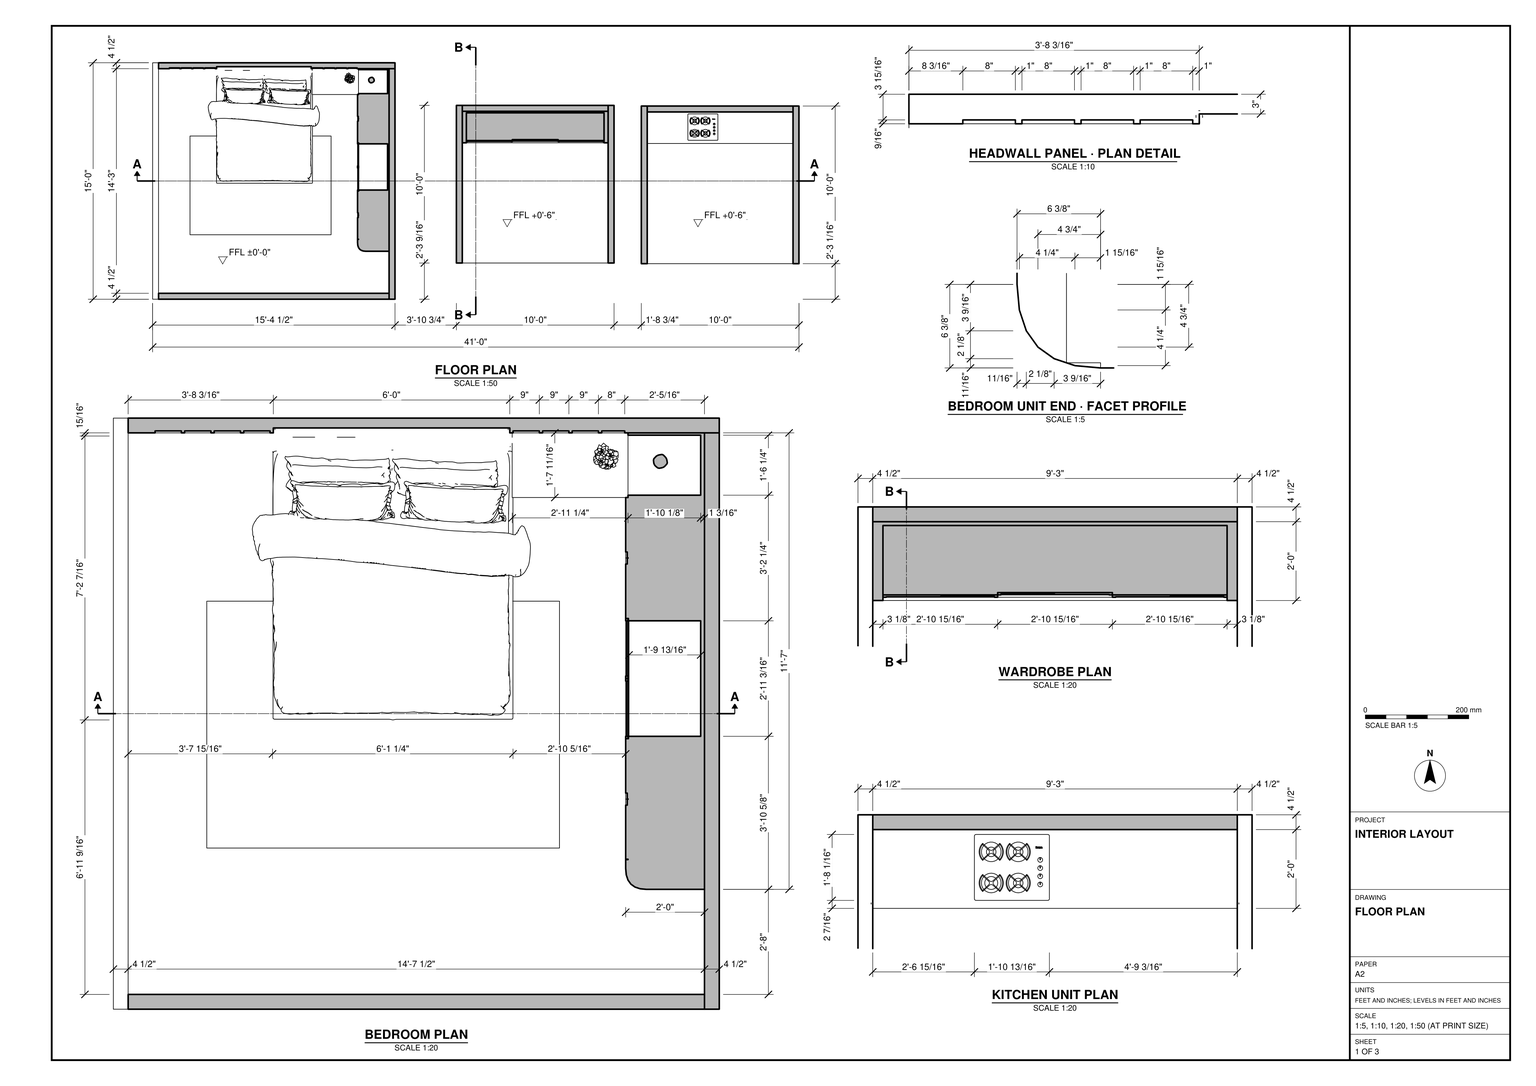
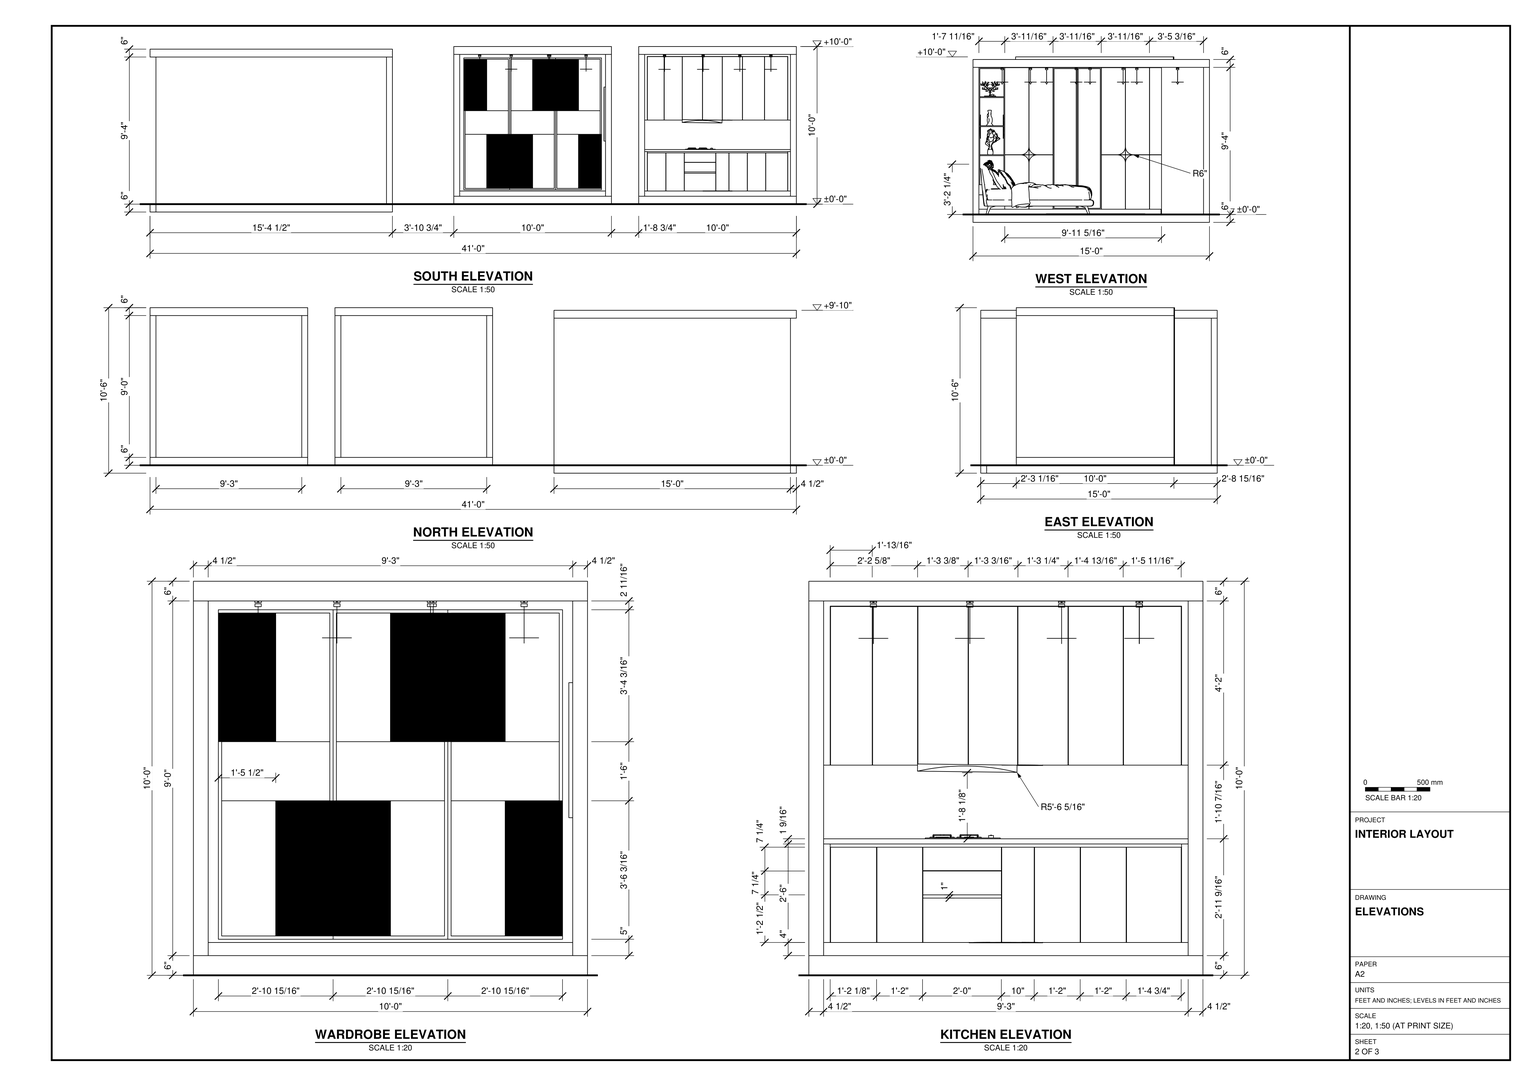
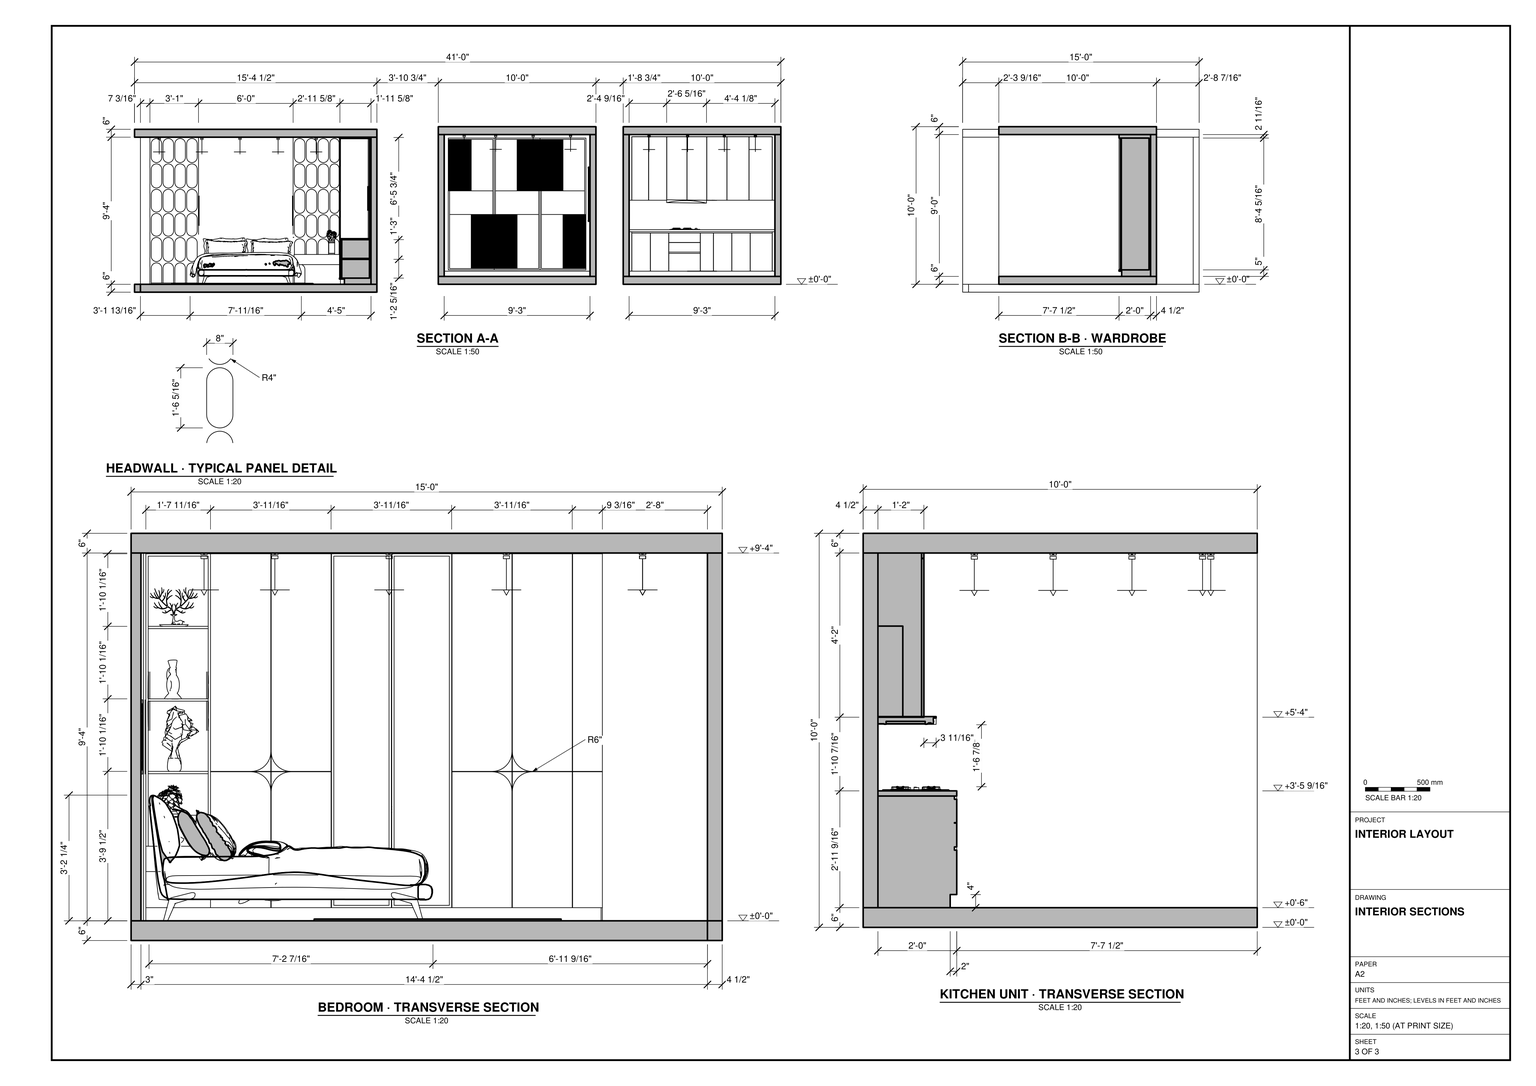
Build the interior layout in SketchUp from task_files/diagram_01.pdf. Work in feet and inches. The overall model is 41'-0" long, 15'-0" deep and 10'-6" high. Use the bedroom finished floor at ±0'-0" as the storey datum. Set the wardrobe and kitchen finished floors at +0'-6"; these are raised bays on the same storey.

Place the 15'-4 1/2" wide bedroom on the left, the wardrobe in the middle and the kitchen on the right. Follow the floor plan for the gaps and setbacks between bays. Form the 4 1/2" walls and 6" floor and overhead slabs, leaving the open faces as drawn. In the bedroom, position the bed against the headwall between the fields of rounded panels. Reproduce the side-wall storage unit with its display shelves, divided fronts and shaped end. Use the enlarged plans and elevations to lay out the wardrobe fronts and the kitchen counter, drawers and upper cabinets. Align the hood with the cooktop.

Decor and loose items, including the rug, cushions, shelf objects, lights and appliances, may be any suitable library components placed as shown. Keep shell elements and individual furniture and joinery pieces in separate groups or components, and use components for repeated parts. Save one SketchUp model as output_files/bedroom_wardrobe_and_kitchen_bays.skp.

# SketchUp Ruby script. Lengths in inches.
U = 1.inch
M = Sketchup.active_model
def pt(a) = Geom::Point3d.new(a.map { |v| v * U })
def face(e, loops, mat)
  f = e.add_face(loops[0].map { |a| pt(a) })
  loops[1..].each { |l| e.add_face(l.map { |a| pt(a) }).erase! }
  f.material = f.back_material = mat if mat
  f
end
# faces: each face lists its corners as indices into pts; further lists are holes
def faces(e, pts, list, mat = nil) = list.each { |f| face(e, (f[0].is_a?(Array) ? f : [f]).map { |l| l.map { |i| pts[i] } }, mat) }
# xy, xz, yz: faces in a plane at the given z, y or x. An outline is a flat list of corners, or four numbers for a rectangle; further outlines are holes
def ring(l) = l.size == 4 ? [[l[0], l[1]], [l[2], l[1]], [l[2], l[3]], [l[0], l[3]]] : l.each_slice(2).to_a
def flat(e, list, mat, &to3) = list.each { |f| face(e, (f[0].is_a?(Array) ? f : [f]).map { |l| ring(l).map { |u, v| to3.(u, v) } }, mat) }
def xy(e, z, list, mat = nil) = flat(e, list, mat) { |x, y| [x, y, z] }
def xz(e, y, list, mat = nil) = flat(e, list, mat) { |x, z| [x, y, z] }
def yz(e, x, list, mat = nil) = flat(e, list, mat) { |y, z| [x, y, z] }
def lines(e, pts, list) = list.each { |a, b| e.add_line(pt(pts[a]), pt(pts[b])) }
# prism: a flat outline (further loops are holes) pulled along v
def prism(e, loops, v, mat = nil)
  f = face(e, loops, mat); d = Geom::Vector3d.new(v.map { |x| x * U })
  f.pushpull(f.normal.samedirection?(d) ? d.length : -d.length)
end
def box(e, o, s, mat = nil) = prism(e, [[o, [o[0] + s[0], o[1], o[2]], [o[0] + s[0], o[1] + s[1], o[2]], [o[0], o[1] + s[1], o[2]]]], [0, 0, s[2]], mat)
def at(x, y, z, deg = 0) = Geom::Transformation.translation(pt([x, y, z])) * Geom::Transformation.rotation(ORIGIN, Z_AXIS, deg.degrees)
def axes(o, x, y, z) = Geom::Transformation.new([*x, 0, *y, 0, *z, 0, *pt(o).to_a, 1])
def part(name) = M.definitions.add(name)
# library, detail: a bought-in or finely detailed component or shape, given as its bounding box
def library(name, o, s) = part(name).tap { |d| box(d.entities, o, s) }
def detail(e, o, s) = box(e.add_group.entities, o, s)
def put(e, d, t, mat = nil) = e.add_instance(d, t).tap { |i| i.material = mat if mat }
def group(e, t, mat = nil) = e.add_group.tap { |g| g.transformation = t; g.material = mat if mat }.entities
root = M.entities
M.materials.add("Oak Veneered MDF (VY2JTJ)").color = [209, 167, 120]
M.materials.add("Oak Veneered MDF (Z561KV)").color = [209, 167, 120]
M.materials.add("Sublime-3029-Pacifique-Glamour-or-Glamorous-Pacific-4K").color = [0, 52, 63]
M.materials.add("Teddy_BookCover").color = [245, 235, 215]
M.materials.add("Teddy_HairLight").color = [51, 36, 26]
M.materials.add("[Color M00]").color = [255, 255, 255]
M.materials["[Color M00]"].alpha = 0.43
M.materials.add("[Color M00]1").color = [255, 255, 255]
M.materials.add("[Color M09]").color = [0, 0, 0]
M.materials.add("[Translucent Glass Gray]").color = [128, 128, 128]
M.materials["[Translucent Glass Gray]"].alpha = 0.5
c1 = library("Спалня Венид",[0.07,-0.07,0],[84.71,86.8,39])
c2 = part("Area rug")
box(c2.entities,[0,0,0],[55.12,78.74,0.39])
c3 = part("Group56\#1")
p = [[0,0,0],[0,0,-43.71],[-13.13,0,-43.71],[85.5,-56,0],[-85.5,-56,0],[85.5,56,0],
  [85.5,0,0],[-85.5,56,0],[13.13,0,-43.71],[-85.5,0,0],[0,0,-70.75]]
lines(c3.entities,p,[[0,1],[1,2],[3,4],[5,6],[7,5],[1,8],[9,0],[0,6],[8,10],[4,9],[6,3],[2,10],
  [9,7]])
c4 = part("Rectangle Light")
put(c4.entities,c3,at(0,0,0))
c5 = library("Interior Props 221 030",[-2.57,-3.63,-0.04],[5.13,7.27,11.89])
c6 = library("Decorative Jar 83-09",[-5.58,-3.02,0],[11.21,6.04,13.74])
c7 = library("Decorative Deer 97-30",[-7.23,-2.03,0],[14.46,4,11.8125])
c8 = library("Interior Plant 273 003 001",[-15.3,-29.38,0],[45.32,44.44,78.66])
c9 = library("Potted Basil 50-07",[-3.85,-3.53,0.03],[7.56,8,18.65])
c10 = library("2-TABLE DE CUISSON CLC2",[-11.42,-10.04,0],[22.84,20.08,1.26])
c11 = library("5-HOTTE ASPIRANTE CLC2",[-15.16,-17.72,-0.29],[30.34,17.72,30.09])
c12 = library("Group\#2",[0,0,0],[180,4.5,112])
c13 = library("Group\#4",[-10.5625,9.18,0],[58.5625,139.01,111.76])
c14 = library("Group\#28",[-3.45,-3.45,-12.01],[8.9,8.9,12.86])
c15 = part("Group\#31")
box(c15.entities,[0,0,0],[4.5,120,108])
c16 = library("Group\#35",[-1.43,0,0],[36.36,0.71,100.34])
c17 = library("Group\#36",[-1.43,0,0],[36.36,0.71,100.34])
c18 = library("Group\#34",[0,0,0],[34.93,0.71,100.34])
c19 = library("Group\#46",[-0.5,-0.5,-0.1],[112,2,0.2])
c20 = library("Group\#45",[-0.5,-0.5,-0.1],[112,2,0.2])
prism(root,[[[376.51,147.05,12],[376.51,142.55,12],[376.51,142.55,47.57],[376.51,142.55,70],[376.51,142.55,120],[376.51,147.05,120]]],[111,0,0])
yz(root,156.35,[[83.1,10.71,99.92,117.06],[101.45,10.71,118.27,117.06]],"[Translucent Glass Gray]")
put(root,c1,at(42.23,88.15,6))
put(root,c2,axes([135.84,49.07,6],[0,1.364,0],[-1.364,0,0],[0,0,1.364]))
put(root,c4,axes([4.5,90,62],[0,-1,0],[0,0,-1],[-1,0,0]))
put(root,c5,at(163.96,167.38,73.59,-68.8))
put(root,c6,at(167.45,165.42,28.71,-90))
put(root,c7,at(162.8,166.98,95.68,-90))
put(root,c8,axes([166.6,166.83,51.5],[0.253,0,0],[0,0.253,0],[0,0,0.253]))
put(root,c9,at(150.05,167.93,28.71))
put(root,c10,at(418.88,131.03,47.57))
put(root,c11,axes([420.23,142.55,67.99],[0.99919,0,0],[0,1,0],[0,0,1]))
g1 = group(root,at(180,0,6),"Teddy_BookCover")
box(g1,[0,0,0],[4.5,175.5,112])
put(root,c12,at(4.5,175.5,6),"Teddy_BookCover")
put(root,c13,at(132,27.31,6),"Sublime-3029-Pacifique-Glamour-or-Glamorous-Pacific-4K")
g2 = group(root,at(157.03,83.1,25.71),"Oak Veneered MDF (Z561KV)")
prism(g2,[[[0,0,14.29],[0,15.59,14.29],[0,15.62,13.99],[0,15.7,13.74],[0,15.84,13.54],[0,16.04,13.4],[0,16.29,13.32],[0,16.6,13.29],[0,18.58,13.29],[0,18.89,13.32],[0,19.14,13.4],[0,19.34,13.54],[0,19.48,13.74],[0,19.5625,13.99],[0,19.59,14.29],[0,35.18,14.29],[0,35.18,0],[0,0,0]]],[0.71,0,0])
g3 = group(root,at(157.03,83.1,10.71),"Oak Veneered MDF (Z561KV)")
prism(g3,[[[0,0,14.29],[0,15.59,14.29],[0,15.62,13.99],[0,15.7,13.74],[0,15.84,13.54],[0,16.04,13.4],[0,16.29,13.32],[0,16.59,13.29],[0,18.59,13.29],[0,18.89,13.32],[0,19.14,13.4],[0,19.34,13.54],[0,19.48,13.74],[0,19.5625,13.99],[0,19.59,14.29],[0,35.18,14.29],[0,35.18,0],[0,0,0]]],[0.71,0,0])
g4 = group(root,at(4.5,0,6),"Teddy_BookCover")
box(g4,[0,0,0],[175.5,4.5,112])
g5 = group(root,at(0,0,118))
box(g5,[0,0,0],[184.5,180,6])
g6 = group(root,at(4.5,0,0),"Teddy_BookCover")
xy(g6,0,[[-4.5,0,0,180],[0,0,180,4.5],[0,4.5,180,180]])
xy(g6,6,[[-4.5,0,0,180],[0,0,180,4.5],[0,4.5,180,180]])
xz(g6,0,[[-4.5,0,0,6],[0,0,180,6]])
xz(g6,4.5,[[0,0,180,6]])
xz(g6,180,[[-4.5,0,0,6],[0,0,180,6]])
yz(g6,-4.5,[[0,0,180,6]])
yz(g6,0,[[0,0,4.5,6],[4.5,0,180,6]])
yz(g6,180,[[0,0,4.5,6],[4.5,0,180,6]])
put(root,c14,at(137.28,156.78,117.15))
put(root,c14,at(137.28,135.22,117.15))
put(root,c14,at(137.28,100.41,117.15))
put(root,c14,at(137.28,64.72,117.15))
put(root,c14,at(137.28,23.22,117.15))
put(root,c14,at(17.78,23.22,117.15))
put(root,c14,at(17.78,156.78,117.15))
put(root,c14,at(17.78,122.97,117.15))
put(root,c14,at(17.78,89.91,117.15))
put(root,c14,at(17.78,54.28,117.15))
put(root,c14,at(108.28,156.78,117.15))
put(root,c14,at(79.28,156.78,117.15))
put(root,c14,at(50.28,156.78,117.15))
put(root,c14,at(50.28,23.28,117.15))
put(root,c14,at(108.28,23.28,117.15))
put(root,c14,at(79.28,23.28,117.15))
g7 = group(root,at(231.24,27.55,6))
box(g7,[0,0,0],[120,120,6])
put(root,c15,at(346.74,27.55,12))
put(root,c15,at(231.24,27.55,12))
g8 = group(root,at(235.74,143.05,12))
box(g8,[0,0,0],[111,4.5,108])
put(root,c16,at(238.84,120.05,16.98),"Oak Veneered MDF (Z561KV)")
put(root,c17,axes([308.7,120.76,16.98],[-1,0,0],[0,1,0],[0,0,1]),"Oak Veneered MDF (Z561KV)")
put(root,c18,at(308.7,120.05,16.98),"Oak Veneered MDF (Z561KV)")
g9 = group(root,at(235.74,119.05,12))
xy(g9,0,[[0,2,111,24]])
xy(g9,4,[[0,0,111,2]])
xy(g9,4.98,[[3.1,0,107.9,1],[3.1,1,107.9,22.83]])
xy(g9,105.32,[[3.1,0,107.9,22.83]],"Teddy_BookCover")
xy(g9,108,[[0,0,111,24]])
xz(g9,0,[[[0,4,111,108],[3.1,4.98,107.9,105.32]]],"Teddy_BookCover")
xz(g9,2,[[0,0,111,4]],"Teddy_BookCover")
xz(g9,22.83,[[3.1,4.98,107.9,105.32]])
xz(g9,24,[[0,0,111,108]])
yz(g9,0,[[2,0,2,4,0,4,0,108,24,108,24,0]])
yz(g9,3.1,[[0,4.98,22.83,105.32]],"Teddy_BookCover")
yz(g9,107.9,[[0,4.98,22.83,105.32]],"Teddy_BookCover")
yz(g9,111,[[2,0,24,0,24,108,0,108,0,4,2,4]])
g10 = group(root,at(231.24,27.55,120))
box(g10,[0,0,0],[120,120,6])
g11 = group(root,at(345.56,62.86,54),"Teddy_HairLight")
xy(g11,0,[[0,0,1.18,36]])
xy(g11,0.71,[[0,0.71,0.12,35.29]])
xy(g11,40.42,[[0,0.71,0.12,35.29]])
xy(g11,41.125,[[0,0,1.18,36]])
xz(g11,0,[[0,0,1.18,41.125]])
xz(g11,0.71,[[0,0.71,0.12,40.42]])
xz(g11,35.29,[[0,0.71,0.12,40.42]])
xz(g11,36,[[0,0,1.18,41.125]])
yz(g11,0,[[[0,0,36,41.125],[0.71,0.71,35.29,40.42]]])
yz(g11,0.12,[[0.71,0.71,35.29,40.42]])
yz(g11,1.18,[[0,0,36,41.125]])
put(root,c14,at(249.93,102.97,119.15))
put(root,c14,at(330.93,102.97,119.15))
put(root,c14,at(273.93,102.97,119.15))
put(root,c14,at(302.43,102.97,119.15))
put(root,c14,at(330.93,78.97,119.15))
put(root,c14,at(249.93,78.97,119.15))
put(root,c14,at(330.93,54.97,119.15))
put(root,c14,at(249.93,54.97,119.15))
put(root,c14,at(330.93,30.97,119.15))
put(root,c14,at(249.93,30.97,119.15))
put(root,c14,at(273.93,30.97,119.15))
put(root,c14,at(303.25,30.97,119.15))
g12 = group(root,at(372.01,27.05,6))
box(g12,[0,0,0],[120,120,6])
g13 = group(root,at(487.51,27.05,12))
box(g13,[0,0,0],[4.5,120,108])
g14 = group(root,at(376.51,118.55,12),"Teddy_BookCover")
xy(g14,0,[[0,2,111,24]])
xy(g14,4,[[0,0,0,1,111,1,111,0,109,0,109,0.71,108.88,0.71,108.88,0,92.24,0,92.24,0.71,92.12,0.71,92.12,0,78.24,0,78.24,0.71,78.12,0.71,78.12,0,64.24,0,64.24,0.71,64.12,0.71,64.12,0,54.24,0,54.24,0.71,54.12,0.71,54.12,0,30.24,0,30.24,0.71,30.12,0.71,30.12,0,16.24,0,16.24,0.71,16.12,0.71,16.12,0,2.12,0,2.12,0.71,2,0.71,2,0]])
xy(g14,17.52,[[30.24,0,54.12,0.71]])
xy(g14,18.51,[[30.24,0,54.12,0.71]])
xy(g14,25.76,[[30.24,0,54.12,0.71]])
xy(g14,25.88,[[30.24,0,54.12,0.71]])
xy(g14,33.02,[[2.12,0,16.12,0.71],[16.24,0,30.12,0.71],[30.24,0,54.12,0.71],[54.24,0,64.12,0.71],[64.24,0,78.12,0.71],
  [78.24,0,92.12,0.71],[92.24,0,108.88,0.71]])
xy(g14,34,[[0,0,0,24,111,24,111,0,109,0,109,0.71,2,0.71,2,0],[2,0,109,0.71]])
xy(g14,35.57,[[0,0,111,24]],"[Color M00]1")
xz(g14,0,[[0,4,2,34],[2.12,4,16.12,33.02],[16.24,4,30.12,33.02],[30.24,4,54.12,17.52],[54.24,4,64.12,33.02],
  [78.24,4,92.12,33.02],[92.24,4,108.88,33.02],[109,4,111,34],[30.24,18.51,54.12,25.76],[30.24,25.88,54.12,33.02]])
xz(g14,0,[[64.24,4,78.12,33.02]],"Teddy_BookCover")
xz(g14,0,[[0,34,111,35.57]],"[Color M00]1")
xz(g14,0.71,[[2,4,2.12,33.02],[16.12,4,16.24,33.02],[30.12,4,30.24,33.02],[54.12,4,54.24,33.02],[64.12,4,64.24,33.02],
  [78.12,4,78.24,33.02],[92.12,4,92.24,33.02],[108.88,4,109,33.02],[30.24,25.76,54.12,25.88]])
xz(g14,0.71,[[30.24,17.52,54.12,18.51],[2,33.02,109,34]],"[Color M09]")
xz(g14,2,[[0,0,111,4]])
xz(g14,24,[[0,0,111,34],[0,34,111,35.57]])
yz(g14,0,[[2,0,2,4,0,4,0,34,24,34,24,0],[0,34,24,35.57]])
yz(g14,2,[[0,4,0.71,33.02],[0,33.02,0.71,34]])
yz(g14,2.12,[[0,4,0.71,33.02]])
yz(g14,16.12,[[0,4,0.71,33.02]])
yz(g14,16.24,[[0,4,0.71,33.02]])
yz(g14,30.12,[[0,4,0.71,33.02]])
yz(g14,30.24,[[0,4,0.71,17.52],[0,18.51,0.71,25.76],[0,25.88,0.71,33.02]])
yz(g14,54.12,[[0,4,0.71,17.52],[0,18.51,0.71,25.76],[0,25.88,0.71,33.02]])
yz(g14,54.24,[[0,4,0.71,33.02]])
yz(g14,64.12,[[0,4,0.71,33.02]])
yz(g14,64.24,[[0,4,0.71,33.02]])
yz(g14,78.12,[[0,4,0.71,33.02]])
yz(g14,78.24,[[0,4,0.71,33.02]])
yz(g14,92.12,[[0,4,0.71,33.02]])
yz(g14,92.24,[[0,4,0.71,33.02]])
yz(g14,108.88,[[0,4,0.71,33.02]])
yz(g14,109,[[0,4,0.71,33.02],[0,33.02,0.71,34]])
yz(g14,111,[[2,0,24,0,24,34,0,34,0,4,2,4]])
yz(g14,111,[[0,34,24,35.57]],"[Color M00]")
put(g14,c19,at(0,1,4))
g15 = group(root,at(376.51,128.55,70),"Oak Veneered MDF (VY2JTJ)")
xy(g15,0,[[0,0.71,111,13]])
xy(g15,0,[[0,0,2,0.71],[2.12,0,14.8,0.71],[14.92,0,20.03,0.71],[20.03,0,28.6,0.71],[28.72,0,37.82,0.71],
  [37.82,0,43.99,0.71],[44.11,0,55.62,0.71],[55.62,0,59.06,0.71],[59.18,0,59.18,0.71,73.41,0.71,74.41,0],[74.41,0,73.41,0.71,74.41,0.71],
  [74.53,0,91.21,0.71],[91.32,0,108.88,0.71],[109,0,111,0.71]],"Oak Veneered MDF (VY2JTJ)")
xy(g15,48.31,[[2.12,0,14.8,0.71],[14.92,0,20.03,0.71],[20.03,0,28.6,0.71],[28.72,0,37.82,0.71],[37.82,0,43.99,0.71],
  [44.11,0,55.62,0.71],[55.62,0,59.06,0.71],[59.18,0,74.41,0,73.41,0.71,59.18,0.71],[74.41,0,74.41,0.71,73.41,0.71],[74.53,0,91.21,0.71],
  [91.32,0,108.88,0.71]],"Oak Veneered MDF (VY2JTJ)")
xy(g15,48.43,[[108.88,0,109,0.71]])
xy(g15,48.43,[[2,0,108.88,0.71]],"Oak Veneered MDF (VY2JTJ)")
xy(g15,50,[[0,0,111,0.71],[0,0.71,111,14]],"Oak Veneered MDF (VY2JTJ)")
xz(g15,0,[[0,0,2,0,2,48.43,109,48.43,109,0,111,0,111,50,0,50],[2.12,0,14.8,48.31],[14.92,0,28.6,48.31],[28.72,0,43.99,48.31],[44.11,0,59.06,48.31],
  [59.18,0,74.41,48.31],[74.53,0,91.21,48.31],[91.32,0,108.88,48.31]],"Oak Veneered MDF (VY2JTJ)")
xz(g15,0.71,[[2,0,2.12,48.31],[108.88,0,109,48.43]])
xz(g15,0.71,[[0,0,0,50,111,50,111,0,109,0,109,48.43,2,48.43,2,0],[2.12,0,14.8,48.31],[14.8,0,14.92,48.31],[14.92,0,20.03,48.31],[20.03,0,28.6,48.31],
  [28.6,0,28.72,48.31],[28.72,0,37.82,48.31],[37.82,0,43.99,48.31],[43.99,0,44.11,48.31],[44.11,0,55.62,48.31],
  [55.62,0,59.06,48.31],[59.06,0,59.18,48.31],[59.18,0,73.41,48.31],[73.41,0,74.41,48.31],[74.41,0,74.53,48.31],
  [74.53,0,91.21,48.31],[91.32,0,108.88,48.31],[2,48.31,108.88,48.43]],"Oak Veneered MDF (VY2JTJ)")
xz(g15,14,[[0,0,111,50]])
yz(g15,0,[[0.71,0,14,50]])
yz(g15,0,[[0,0,0.71,50]],"Oak Veneered MDF (VY2JTJ)")
yz(g15,2,[[0,0,0.71,48.31],[0,48.31,0.71,48.43]],"Oak Veneered MDF (VY2JTJ)")
yz(g15,2.12,[[0,0,0.71,48.31]])
yz(g15,14.8,[[0,0,0.71,48.31]],"Oak Veneered MDF (VY2JTJ)")
yz(g15,14.92,[[0,0,0.71,48.31]],"Oak Veneered MDF (VY2JTJ)")
yz(g15,28.6,[[0,0,0.71,48.31]],"Oak Veneered MDF (VY2JTJ)")
yz(g15,28.72,[[0,0,0.71,48.31]],"Oak Veneered MDF (VY2JTJ)")
yz(g15,43.99,[[0,0,0.71,48.31]],"Oak Veneered MDF (VY2JTJ)")
yz(g15,44.11,[[0,0,0.71,48.31]],"Oak Veneered MDF (VY2JTJ)")
yz(g15,59.06,[[0,0,0.71,48.31]],"Oak Veneered MDF (VY2JTJ)")
yz(g15,59.18,[[0,0,0.71,48.31]],"Oak Veneered MDF (VY2JTJ)")
yz(g15,74.41,[[0,0,0.71,48.31]],"Oak Veneered MDF (VY2JTJ)")
yz(g15,74.53,[[0,0,0.71,48.31]],"Oak Veneered MDF (VY2JTJ)")
yz(g15,91.21,[[0,0,0.71,48.31]])
yz(g15,91.32,[[0,0,0.71,48.31]],"Oak Veneered MDF (VY2JTJ)")
yz(g15,108.88,[[0,0,0.71,48.31]],"Oak Veneered MDF (VY2JTJ)")
yz(g15,109,[[0,0,0.71,48.43]],"Oak Veneered MDF (VY2JTJ)")
yz(g15,111,[[0.71,0,14,50]])
yz(g15,111,[[0,0,0.71,50]],"Oak Veneered MDF (VY2JTJ)")
p = [[74.41,0,0],[74.41,0,48.31],[73.41,0.71,48.31],[73.41,0.71,0]]
faces(g15,p,[[0,1,2,3]])
put(g15,c20,at(0,13,0))
g16 = group(root,at(372.01,27.05,120))
box(g16,[0,0,0],[120,120,6])
g17 = group(root,at(372.01,27.05,12))
box(g17,[0,0,0],[4.5,120,108])
put(root,c14,at(390.67,112.2,119))
put(root,c14,at(420.04,112.2,119))
put(root,c14,at(447.98,112.2,119))
put(root,c14,at(471.6,112.2,119))
put(root,c14,at(390.67,88.2,119))
put(root,c14,at(390.67,64.2,119))
put(root,c14,at(390.67,40.2,119))
put(root,c14,at(471.67,64.2,119))
put(root,c14,at(471.67,88.2,119))
put(root,c14,at(471.67,40.2,119))
put(root,c14,at(447.98,42.7,119))
put(root,c14,at(420.04,42.7,119))
